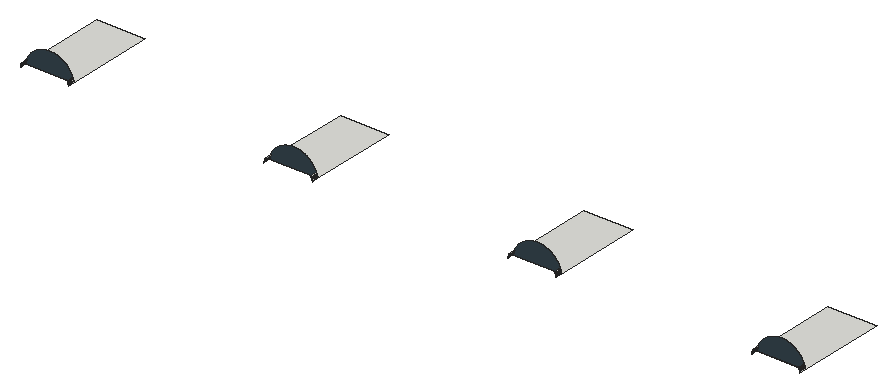
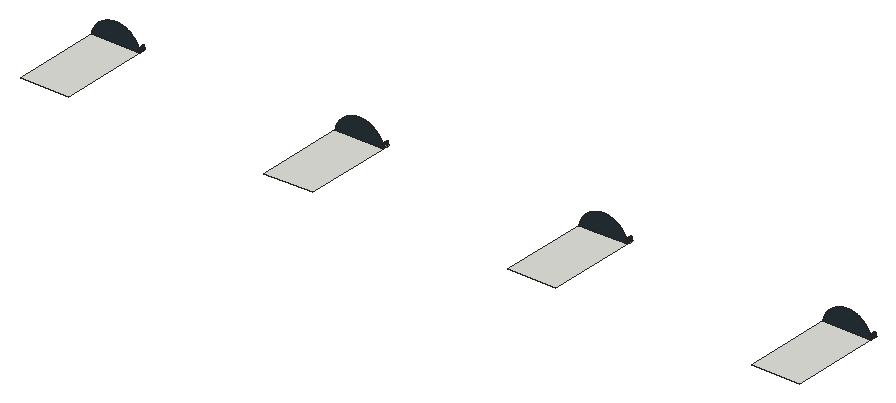
# SketchUp Ruby script. Lengths in inches.
U = 1.inch
M = Sketchup.active_model
def pt(a) = Geom::Point3d.new(a.map { |v| v * U })
def face(e, loops, mat)
  f = e.add_face(loops[0].map { |a| pt(a) })
  loops[1..].each { |l| e.add_face(l.map { |a| pt(a) }).erase! }
  f.material = f.back_material = mat if mat
  f
end
# faces: each face lists its corners as indices into pts; further lists are holes
def faces(e, pts, list, mat = nil) = list.each { |f| face(e, (f[0].is_a?(Array) ? f : [f]).map { |l| l.map { |i| pts[i] } }, mat) }
# xy, xz, yz: faces in a plane at the given z, y or x. An outline is a flat list of corners, or four numbers for a rectangle; further outlines are holes
def ring(l) = l.size == 4 ? [[l[0], l[1]], [l[2], l[1]], [l[2], l[3]], [l[0], l[3]]] : l.each_slice(2).to_a
def flat(e, list, mat, &to3) = list.each { |f| face(e, (f[0].is_a?(Array) ? f : [f]).map { |l| ring(l).map { |u, v| to3.(u, v) } }, mat) }
def xy(e, z, list, mat = nil) = flat(e, list, mat) { |x, y| [x, y, z] }
def xz(e, y, list, mat = nil) = flat(e, list, mat) { |x, z| [x, y, z] }
def yz(e, x, list, mat = nil) = flat(e, list, mat) { |y, z| [x, y, z] }
def lines(e, pts, list) = list.each { |a, b| e.add_line(pt(pts[a]), pt(pts[b])) }
# prism: a flat outline (further loops are holes) pulled along v
def prism(e, loops, v, mat = nil)
  f = face(e, loops, mat); d = Geom::Vector3d.new(v.map { |x| x * U })
  f.pushpull(f.normal.samedirection?(d) ? d.length : -d.length)
end
def box(e, o, s, mat = nil) = prism(e, [[o, [o[0] + s[0], o[1], o[2]], [o[0] + s[0], o[1] + s[1], o[2]], [o[0], o[1] + s[1], o[2]]]], [0, 0, s[2]], mat)
def at(x, y, z, deg = 0) = Geom::Transformation.translation(pt([x, y, z])) * Geom::Transformation.rotation(ORIGIN, Z_AXIS, deg.degrees)
def axes(o, x, y, z) = Geom::Transformation.new([*x, 0, *y, 0, *z, 0, *pt(o).to_a, 1])
def part(name) = M.definitions.add(name)
# library, detail: a bought-in or finely detailed component or shape, given as its bounding box
def library(name, o, s) = part(name).tap { |d| box(d.entities, o, s) }
def detail(e, o, s) = box(e.add_group.entities, o, s)
def put(e, d, t, mat = nil) = e.add_instance(d, t).tap { |i| i.material = mat if mat }
def group(e, t, mat = nil) = e.add_group.tap { |g| g.transformation = t; g.material = mat if mat }.entities
root = M.entities
M.materials.add("1480 AP K099 Starless Night-N").color = [54, 68, 77]
xy(root,235.48,[[175,224.6875,175.125,229.25],[619,224.6875,619.125,229.25],[1063,224.6875,1063.125,229.25],[1507,224.6875,1507.125,229.25],[175.125,236.25,263,398.125],
  [619.125,236.25,707,398.125],[1063.125,236.25,1151,398.125],[1507.125,236.25,1595,398.125]])
xz(root,236.25,[[175.125,235.48,263,235.48,262.87,236.07,262.73,236.67,262.58,237.26,262.42,237.85,262.08,239.03,261.9,239.61,261.71,240.19,261.31,241.35,261.1,241.92,260.65,243.06,260.17,244.18,259.92,244.74,259.66,245.3,259.39,245.85,259.12,246.39,258.84,246.9375,258.55,247.48,258.26,248.01,257.64,249.07,257.33,249.59,257,250.11,256.67,250.625,256.33,251.13,255.99,251.64,255.64,252.14,255.28,252.63,254.91,253.125,254.54,253.61,254.16,254.09,253.78,254.5625,253.39,255.03,252.99,255.5,252.58,255.96,251.76,256.86,251.34,257.3,250.91,257.74,250.47,258.17,249.59,259.01,249.14,259.42,248.68,259.83,248.22,260.23,247.75,260.625,247.28,261.01,246.8,261.39,246.3125,261.77,245.82,262.13,245.33,262.49,244.83,262.85,244.33,263.2,243.82,263.54,243.31,263.87,242.79,264.2,242.27,264.52,241.75,264.83,241.22,265.14,240.68,265.43,240.15,265.72,239.6,266.01,239.06,266.28,238.51,266.55,237.96,266.8125,237.4,267.07,236.84,267.3125,236.28,267.55,235.14,268.01,234.57,268.22,233.99,268.43,233.42,268.63,232.84,268.82,232.25,269,231.67,269.18,231.08,269.35,230.49,269.51,229.9,269.66,229.3,269.81,228.71,269.94,228.11,270.07,227.51,270.1875,226.91,270.3,226.3,270.4,225.7,270.5,225.1,270.59,223.27,270.8,222.05,270.9,220.83,270.96,219.61,271,218.38,271,217.77,270.98,217.15,270.96,216.53,270.93,215.92,270.89,215.3,270.85,214.6875,270.79,214.08,270.73,213.46,270.66,212.85,270.58,212.24,270.49,211.02,270.29,210.42,270.17,209.8125,270.05,209.21,269.92,208.61,269.78,207.41,269.48,206.23,269.14,205.05,268.78,204.46,268.58,203.88,268.375,203.3,268.16,202.73,267.94,202.15,267.72,201.58,267.48,201.02,267.24,200.45,266.99,199.89,266.73,199.34,266.46,198.79,266.1875,198.24,265.91,197.69,265.62,196.61,265.02,196.08,264.7,195.55,264.39,194.51,263.73,194,263.39,193.49,263.04,192.98,262.68,192.48,262.32,191.99,261.96,191.01,261.2,190.53,260.8125,190.06,260.42,189.59,260.02,189.13,259.61,188.67,259.19,187.77,258.35,186.9,257.48,186.47,257.03,186.05,256.58,185.64,256.125,185.23,255.66,184.82,255.2,184.43,254.72,184.04,254.25,183.65,253.76,182.91,252.78,182.19,251.78,181.84,251.27,181.5,250.76,181.16,250.24,180.84,249.72,180.2,248.66,179.6,247.58,179.31,247.04,179.02,246.49,178.75,245.94,178.48,245.38,178.22,244.83,177.97,244.26,177.72,243.7,177.48,243.13,177.25,242.56,177.03,241.98,176.61,240.82,176.41,240.24,176.22,239.65,176.04,239.06,175.87,238.47,175.7,237.875,175.55,237.28,175.4,236.68,175.26,236.08],[619.125,235.48,707,235.48,706.87,236.07,706.73,236.67,706.58,237.26,706.42,237.85,706.08,239.03,705.9,239.61,705.71,240.19,705.31,241.35,705.1,241.92,704.65,243.06,704.17,244.18,703.92,244.74,703.66,245.3,703.39,245.85,703.12,246.39,702.84,246.9375,702.55,247.48,702.26,248.01,701.64,249.07,701.33,249.59,701,250.11,700.67,250.625,700.33,251.13,699.99,251.64,699.64,252.14,699.28,252.63,698.91,253.125,698.54,253.61,698.16,254.09,697.78,254.5625,697.39,255.03,696.99,255.5,696.58,255.96,695.76,256.86,695.34,257.3,694.91,257.74,694.47,258.17,693.59,259.01,693.14,259.42,692.68,259.83,692.22,260.23,691.75,260.625,691.28,261.01,690.8,261.39,690.3125,261.77,689.82,262.13,689.33,262.49,688.83,262.85,688.33,263.2,687.82,263.54,687.31,263.87,686.79,264.2,686.27,264.52,685.75,264.83,685.22,265.14,684.68,265.43,684.15,265.72,683.6,266.01,683.06,266.28,682.51,266.55,681.96,266.8125,681.4,267.07,680.84,267.3125,680.28,267.55,679.14,268.01,678.57,268.22,677.99,268.43,677.42,268.63,676.84,268.82,676.25,269,675.67,269.18,675.08,269.35,674.49,269.51,673.9,269.66,673.3,269.81,672.71,269.94,672.11,270.07,671.51,270.1875,670.91,270.3,670.3,270.4,669.7,270.5,669.1,270.59,667.27,270.8,666.05,270.9,664.83,270.96,663.61,271,662.38,271,661.77,270.98,661.15,270.96,660.53,270.93,659.92,270.89,659.3,270.85,658.6875,270.79,658.08,270.73,657.46,270.66,656.85,270.58,656.24,270.49,655.02,270.29,654.42,270.17,653.8125,270.05,653.21,269.92,652.61,269.78,651.41,269.48,650.23,269.14,649.05,268.78,648.46,268.58,647.88,268.375,647.3,268.16,646.73,267.94,646.15,267.72,645.58,267.48,645.02,267.24,644.45,266.99,643.89,266.73,643.34,266.46,642.79,266.1875,642.24,265.91,641.69,265.62,640.61,265.02,640.08,264.7,639.55,264.39,638.51,263.73,638,263.39,637.49,263.04,636.98,262.68,636.48,262.32,635.99,261.96,635.01,261.2,634.53,260.8125,634.06,260.42,633.59,260.02,633.13,259.61,632.67,259.19,631.77,258.35,630.9,257.48,630.47,257.03,630.05,256.58,629.64,256.125,629.23,255.66,628.82,255.2,628.43,254.72,628.04,254.25,627.65,253.76,626.91,252.78,626.19,251.78,625.84,251.27,625.5,250.76,625.16,250.24,624.84,249.72,624.2,248.66,623.6,247.58,623.31,247.04,623.02,246.49,622.75,245.94,622.48,245.38,622.22,244.83,621.97,244.26,621.72,243.7,621.48,243.13,621.25,242.56,621.03,241.98,620.61,240.82,620.41,240.24,620.22,239.65,620.04,239.06,619.87,238.47,619.7,237.875,619.55,237.28,619.4,236.68,619.26,236.08],[1063.125,235.48,1151,235.48,1150.87,236.07,1150.73,236.67,1150.58,237.26,1150.42,237.85,1150.08,239.03,1149.9,239.61,1149.71,240.19,1149.31,241.35,1149.1,241.92,1148.65,243.06,1148.17,244.18,1147.92,244.74,1147.66,245.3,1147.39,245.85,1147.12,246.39,1146.84,246.9375,1146.55,247.48,1146.26,248.01,1145.64,249.07,1145.33,249.59,1145,250.11,1144.67,250.625,1144.33,251.13,1143.99,251.64,1143.64,252.14,1143.28,252.63,1142.91,253.125,1142.54,253.61,1142.16,254.09,1141.78,254.5625,1141.39,255.03,1140.99,255.5,1140.58,255.96,1139.76,256.86,1139.34,257.3,1138.91,257.74,1138.47,258.17,1137.59,259.01,1137.14,259.42,1136.68,259.83,1136.22,260.23,1135.75,260.625,1135.28,261.01,1134.8,261.39,1134.3125,261.77,1133.82,262.13,1133.33,262.49,1132.83,262.85,1132.33,263.2,1131.82,263.54,1131.31,263.87,1130.79,264.2,1130.27,264.52,1129.75,264.83,1129.22,265.14,1128.68,265.43,1128.15,265.72,1127.6,266.01,1127.06,266.28,1126.51,266.55,1125.96,266.8125,1125.4,267.07,1124.84,267.3125,1124.28,267.55,1123.14,268.01,1122.57,268.22,1121.99,268.43,1121.42,268.63,1120.84,268.82,1120.25,269,1119.67,269.18,1119.08,269.35,1118.49,269.51,1117.9,269.66,1117.3,269.81,1116.71,269.94,1116.11,270.07,1115.51,270.1875,1114.91,270.3,1114.3,270.4,1113.7,270.5,1113.1,270.59,1111.27,270.8,1110.05,270.9,1108.83,270.96,1107.61,271,1106.38,271,1105.77,270.98,1105.15,270.96,1104.53,270.93,1103.92,270.89,1103.3,270.85,1102.6875,270.79,1102.08,270.73,1101.46,270.66,1100.85,270.58,1100.24,270.49,1099.02,270.29,1098.42,270.17,1097.8125,270.05,1097.21,269.92,1096.61,269.78,1095.41,269.48,1094.23,269.14,1093.05,268.78,1092.46,268.58,1091.88,268.375,1091.3,268.16,1090.73,267.94,1090.15,267.72,1089.58,267.48,1089.02,267.24,1088.45,266.99,1087.89,266.73,1087.34,266.46,1086.79,266.1875,1086.24,265.91,1085.69,265.62,1084.61,265.02,1084.08,264.7,1083.55,264.39,1082.51,263.73,1082,263.39,1081.49,263.04,1080.98,262.68,1080.48,262.32,1079.99,261.96,1079.01,261.2,1078.53,260.8125,1078.06,260.42,1077.59,260.02,1077.13,259.61,1076.67,259.19,1075.77,258.35,1074.9,257.48,1074.47,257.03,1074.05,256.58,1073.64,256.125,1073.23,255.66,1072.82,255.2,1072.43,254.72,1072.04,254.25,1071.65,253.76,1070.91,252.78,1070.19,251.78,1069.84,251.27,1069.5,250.76,1069.16,250.24,1068.84,249.72,1068.2,248.66,1067.6,247.58,1067.31,247.04,1067.02,246.49,1066.75,245.94,1066.48,245.38,1066.22,244.83,1065.97,244.26,1065.72,243.7,1065.48,243.13,1065.25,242.56,1065.03,241.98,1064.61,240.82,1064.41,240.24,1064.22,239.65,1064.04,239.06,1063.87,238.47,1063.7,237.875,1063.55,237.28,1063.4,236.68,1063.26,236.08],[1507.125,235.48,1595,235.48,1594.87,236.07,1594.73,236.67,1594.58,237.26,1594.42,237.85,1594.08,239.03,1593.9,239.61,1593.71,240.19,1593.31,241.35,1593.1,241.92,1592.65,243.06,1592.17,244.18,1591.92,244.74,1591.66,245.3,1591.39,245.85,1591.12,246.39,1590.84,246.9375,1590.55,247.48,1590.26,248.01,1589.64,249.07,1589.33,249.59,1589,250.11,1588.67,250.625,1588.33,251.13,1587.99,251.64,1587.64,252.14,1587.28,252.63,1586.91,253.125,1586.54,253.61,1586.16,254.09,1585.78,254.5625,1585.39,255.03,1584.99,255.5,1584.58,255.96,1583.76,256.86,1583.34,257.3,1582.91,257.74,1582.47,258.17,1581.59,259.01,1581.14,259.42,1580.68,259.83,1580.22,260.23,1579.75,260.625,1579.28,261.01,1578.8,261.39,1578.3125,261.77,1577.82,262.13,1577.33,262.49,1576.83,262.85,1576.33,263.2,1575.82,263.54,1575.31,263.87,1574.79,264.2,1574.27,264.52,1573.75,264.83,1573.22,265.14,1572.68,265.43,1572.15,265.72,1571.6,266.01,1571.06,266.28,1570.51,266.55,1569.96,266.8125,1569.4,267.07,1568.84,267.3125,1568.28,267.55,1567.14,268.01,1566.57,268.22,1565.99,268.43,1565.42,268.63,1564.84,268.82,1564.25,269,1563.67,269.18,1563.08,269.35,1562.49,269.51,1561.9,269.66,1561.3,269.81,1560.71,269.94,1560.11,270.07,1559.51,270.1875,1558.91,270.3,1558.3,270.4,1557.7,270.5,1557.1,270.59,1555.27,270.8,1554.05,270.9,1552.83,270.96,1551.61,271,1550.38,271,1549.77,270.98,1549.15,270.96,1548.53,270.93,1547.92,270.89,1547.3,270.85,1546.6875,270.79,1546.08,270.73,1545.46,270.66,1544.85,270.58,1544.24,270.49,1543.02,270.29,1542.42,270.17,1541.8125,270.05,1541.21,269.92,1540.61,269.78,1539.41,269.48,1538.23,269.14,1537.05,268.78,1536.46,268.58,1535.88,268.375,1535.3,268.16,1534.73,267.94,1534.15,267.72,1533.58,267.48,1533.02,267.24,1532.45,266.99,1531.89,266.73,1531.34,266.46,1530.79,266.1875,1530.24,265.91,1529.69,265.62,1528.61,265.02,1528.08,264.7,1527.55,264.39,1526.51,263.73,1526,263.39,1525.49,263.04,1524.98,262.68,1524.48,262.32,1523.99,261.96,1523.01,261.2,1522.53,260.8125,1522.06,260.42,1521.59,260.02,1521.13,259.61,1520.67,259.19,1519.77,258.35,1518.9,257.48,1518.47,257.03,1518.05,256.58,1517.64,256.125,1517.23,255.66,1516.82,255.2,1516.43,254.72,1516.04,254.25,1515.65,253.76,1514.91,252.78,1514.19,251.78,1513.84,251.27,1513.5,250.76,1513.16,250.24,1512.84,249.72,1512.2,248.66,1511.6,247.58,1511.31,247.04,1511.02,246.49,1510.75,245.94,1510.48,245.38,1510.22,244.83,1509.97,244.26,1509.72,243.7,1509.48,243.13,1509.25,242.56,1509.03,241.98,1508.61,240.82,1508.41,240.24,1508.22,239.65,1508.04,239.06,1507.87,238.47,1507.7,237.875,1507.55,237.28,1507.4,236.68,1507.26,236.08]],"1480 AP K099 Starless Night-N")
p = [[175.26,236.25,236.08],[175.26,224.6875,236.08],[175.125,224.6875,235.48],[175.125,229.25,235.48],[175.125,236.25,235.48],[263,236.25,235.48],
  [263,224.6875,235.48],[262.87,224.6875,236.07],[262.87,236.25,236.07],[619.26,236.25,236.08],[619.26,224.6875,236.08],[619.125,224.6875,235.48],
  [619.125,229.25,235.48],[619.125,236.25,235.48],[707,236.25,235.48],[707,224.6875,235.48],[706.87,224.6875,236.07],[706.87,236.25,236.07],
  [1063.26,236.25,236.08],[1063.26,224.6875,236.08],[1063.125,224.6875,235.48],[1063.125,229.25,235.48],[1063.125,236.25,235.48],[1151,236.25,235.48],
  [1151,224.6875,235.48],[1150.87,224.6875,236.07],[1150.87,236.25,236.07],[1507.26,236.25,236.08],[1507.26,224.6875,236.08],[1507.125,224.6875,235.48],
  [1507.125,229.25,235.48],[1507.125,236.25,235.48],[1595,236.25,235.48],[1595,224.6875,235.48],[1594.87,224.6875,236.07],[1594.87,236.25,236.07],
  [175.4,236.25,236.68],[175.4,224.6875,236.68],[262.73,224.6875,236.67],[262.73,236.25,236.67],[619.4,236.25,236.68],[619.4,224.6875,236.68],
  [706.73,224.6875,236.67],[706.73,236.25,236.67],[1063.4,236.25,236.68],[1063.4,224.6875,236.68],[1150.73,224.6875,236.67],[1150.73,236.25,236.67],
  [1507.4,236.25,236.68],[1507.4,224.6875,236.68],[1594.73,224.6875,236.67],[1594.73,236.25,236.67],[175.55,236.25,237.28],[175.55,224.6875,237.28],
  [262.58,224.6875,237.26],[262.58,236.25,237.26],[619.55,236.25,237.28],[619.55,224.6875,237.28],[706.58,224.6875,237.26],[706.58,236.25,237.26],
  [1063.55,236.25,237.28],[1063.55,224.6875,237.28],[1150.58,224.6875,237.26],[1150.58,236.25,237.26],[1507.55,236.25,237.28],[1507.55,224.6875,237.28],
  [1594.58,224.6875,237.26],[1594.58,236.25,237.26],[175.7,236.25,237.875],[175.7,224.6875,237.875],[262.42,224.6875,237.85],[262.42,236.25,237.85],
  [619.7,236.25,237.875],[619.7,224.6875,237.875],[706.42,224.6875,237.85],[706.42,236.25,237.85],[1063.7,236.25,237.875],[1063.7,224.6875,237.875],
  [1150.42,224.6875,237.85],[1150.42,236.25,237.85],[1507.7,236.25,237.875],[1507.7,224.6875,237.875],[1594.42,224.6875,237.85],[1594.42,236.25,237.85],
  [175.87,236.25,238.47],[175.87,224.6875,238.47],[262.25,224.6875,238.44],[262.25,236.25,238.44],[619.87,236.25,238.47],[619.87,224.6875,238.47],
  [706.25,224.6875,238.44],[706.25,236.25,238.44],[1063.87,236.25,238.47],[1063.87,224.6875,238.47],[1150.25,224.6875,238.44],[1150.25,236.25,238.44],
  [1507.87,236.25,238.47],[1507.87,224.6875,238.47],[1594.25,224.6875,238.44],[1594.25,236.25,238.44],[262.08,224.6875,239.03],[262.08,236.25,239.03],
  [706.08,224.6875,239.03],[706.08,236.25,239.03],[1150.08,224.6875,239.03],[1150.08,236.25,239.03],[1594.08,224.6875,239.03],[1594.08,236.25,239.03],
  [176.04,236.25,239.06],[176.04,224.6875,239.06],[620.04,236.25,239.06],[620.04,224.6875,239.06],[1064.04,236.25,239.06],[1064.04,224.6875,239.06],
  [1508.04,236.25,239.06],[1508.04,224.6875,239.06],[261.9,224.6875,239.61],[261.9,236.25,239.61],[705.9,224.6875,239.61],[705.9,236.25,239.61],
  [1149.9,224.6875,239.61],[1149.9,236.25,239.61],[1593.9,224.6875,239.61],[1593.9,236.25,239.61],[176.22,236.25,239.65],[176.22,224.6875,239.65],
  [620.22,236.25,239.65],[620.22,224.6875,239.65],[1064.22,236.25,239.65],[1064.22,224.6875,239.65],[1508.22,236.25,239.65],[1508.22,224.6875,239.65],
  [176.41,236.25,240.24],[176.41,224.6875,240.24],[261.71,224.6875,240.19],[261.71,236.25,240.19],[620.41,236.25,240.24],[620.41,224.6875,240.24],
  [705.71,224.6875,240.19],[705.71,236.25,240.19],[1064.41,236.25,240.24],[1064.41,224.6875,240.24],[1149.71,224.6875,240.19],[1149.71,236.25,240.19],
  [1508.41,236.25,240.24],[1508.41,224.6875,240.24],[1593.71,224.6875,240.19],[1593.71,236.25,240.19],[176.61,236.25,240.82],[176.61,224.6875,240.82],
  [261.51,224.6875,240.77],[261.51,236.25,240.77],[620.61,236.25,240.82],[620.61,224.6875,240.82],[705.51,224.6875,240.77],[705.51,236.25,240.77],
  [1064.61,236.25,240.82],[1064.61,224.6875,240.82],[1149.51,224.6875,240.77],[1149.51,236.25,240.77],[1508.61,236.25,240.82],[1508.61,224.6875,240.82],
  [1593.51,224.6875,240.77],[1593.51,236.25,240.77],[176.82,236.25,241.4],[176.82,224.6875,241.4],[261.31,224.6875,241.35],[261.31,236.25,241.35],
  [620.82,236.25,241.4],[620.82,224.6875,241.4],[705.31,224.6875,241.35],[705.31,236.25,241.35],[1064.82,236.25,241.4],[1064.82,224.6875,241.4],
  [1149.31,224.6875,241.35],[1149.31,236.25,241.35],[1508.82,236.25,241.4],[1508.82,224.6875,241.4],[1593.31,224.6875,241.35],[1593.31,236.25,241.35],
  [261.1,224.6875,241.92],[261.1,236.25,241.92],[705.1,224.6875,241.92],[705.1,236.25,241.92],[1149.1,224.6875,241.92],[1149.1,236.25,241.92],
  [1593.1,224.6875,241.92],[1593.1,236.25,241.92],[177.03,236.25,241.98],[177.03,224.6875,241.98],[621.03,236.25,241.98],[621.03,224.6875,241.98],
  [1065.03,236.25,241.98],[1065.03,224.6875,241.98],[1509.03,236.25,241.98],[1509.03,224.6875,241.98],[260.875,224.6875,242.49],[260.875,236.25,242.49],
  [704.875,224.6875,242.49],[704.875,236.25,242.49],[1148.875,224.6875,242.49],[1148.875,236.25,242.49],[1592.875,224.6875,242.49],[1592.875,236.25,242.49],
  [177.25,236.25,242.56],[177.25,224.6875,242.56],[621.25,236.25,242.56],[621.25,224.6875,242.56],[1065.25,236.25,242.56],[1065.25,224.6875,242.56],
  [1509.25,236.25,242.56],[1509.25,224.6875,242.56],[260.65,224.6875,243.06],[260.65,236.25,243.06],[704.65,224.6875,243.06],[704.65,236.25,243.06],
  [1148.65,224.6875,243.06],[1148.65,236.25,243.06],[1592.65,224.6875,243.06],[1592.65,236.25,243.06],[177.48,236.25,243.13],[177.48,224.6875,243.13],
  [621.48,236.25,243.13],[621.48,224.6875,243.13],[1065.48,236.25,243.13],[1065.48,224.6875,243.13],[1509.48,236.25,243.13],[1509.48,224.6875,243.13]]
faces(root,p,[[0,1,2,3,4],[5,6,7,8],[9,10,11,12,13],[14,15,16,17],[18,19,20,21,22],[23,24,25,26],[27,28,29,30,31],[32,33,34,35],
  [36,37,1,0],[8,7,38,39],[40,41,10,9],[17,16,42,43],[44,45,19,18],[26,25,46,47],[48,49,28,27],[35,34,50,51],
  [52,53,37,36],[39,38,54,55],[56,57,41,40],[43,42,58,59],[60,61,45,44],[47,46,62,63],[64,65,49,48],[51,50,66,67],
  [68,69,53,52],[55,54,70,71],[72,73,57,56],[59,58,74,75],[76,77,61,60],[63,62,78,79],[80,81,65,64],[67,66,82,83],
  [84,85,69,68],[71,70,86,87],[88,89,73,72],[75,74,90,91],[92,93,77,76],[79,78,94,95],[96,97,81,80],[83,82,98,99],
  [87,86,100,101],[91,90,102,103],[95,94,104,105],[99,98,106,107],[108,109,85,84],[110,111,89,88],[112,113,93,92],[114,115,97,96],
  [101,100,116,117],[103,102,118,119],[105,104,120,121],[107,106,122,123],[124,125,109,108],[126,127,111,110],[128,129,113,112],[130,131,115,114],
  [132,133,125,124],[117,116,134,135],[136,137,127,126],[119,118,138,139],[140,141,129,128],[121,120,142,143],[144,145,131,130],[123,122,146,147],
  [148,149,133,132],[135,134,150,151],[152,153,137,136],[139,138,154,155],[156,157,141,140],[143,142,158,159],[160,161,145,144],[147,146,162,163],
  [164,165,149,148],[151,150,166,167],[168,169,153,152],[155,154,170,171],[172,173,157,156],[159,158,174,175],[176,177,161,160],[163,162,178,179],
  [167,166,180,181],[171,170,182,183],[175,174,184,185],[179,178,186,187],[188,189,165,164],[190,191,169,168],[192,193,173,172],[194,195,177,176],
  [181,180,196,197],[183,182,198,199],[185,184,200,201],[187,186,202,203],[204,205,189,188],[206,207,191,190],[208,209,193,192],[210,211,195,194],
  [197,196,212,213],[199,198,214,215],[201,200,216,217],[203,202,218,219],[220,221,205,204],[222,223,207,206],[224,225,209,208],[226,227,211,210]])
